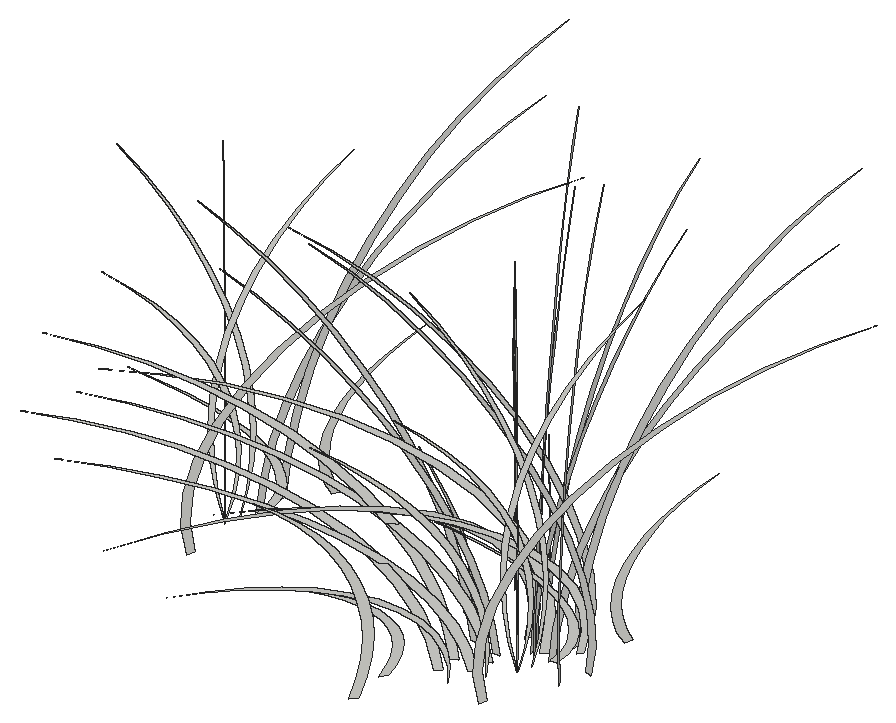
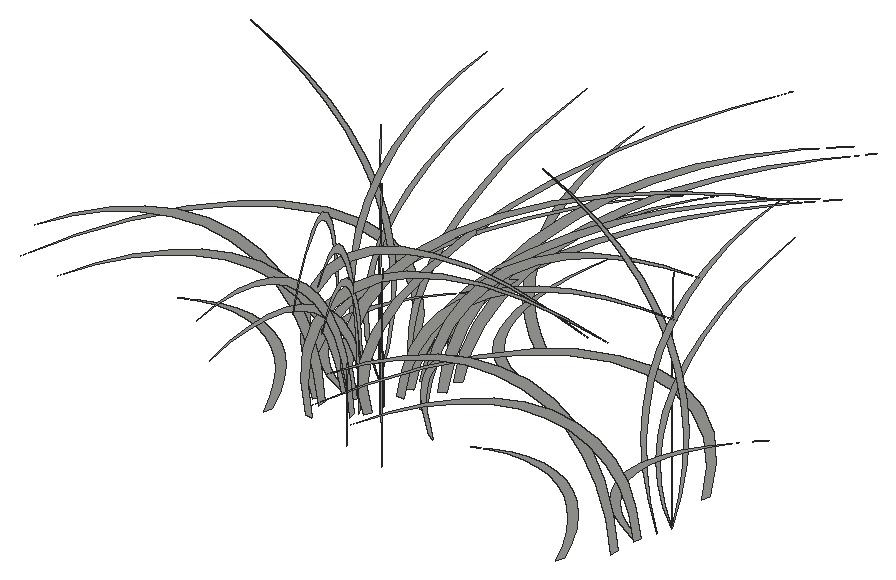
# SketchUp Ruby script. Lengths in inches.
U = 1.inch
M = Sketchup.active_model
def pt(a) = Geom::Point3d.new(a.map { |v| v * U })
def face(e, loops, mat)
  f = e.add_face(loops[0].map { |a| pt(a) })
  loops[1..].each { |l| e.add_face(l.map { |a| pt(a) }).erase! }
  f.material = f.back_material = mat if mat
  f
end
# faces: each face lists its corners as indices into pts; further lists are holes
def faces(e, pts, list, mat = nil) = list.each { |f| face(e, (f[0].is_a?(Array) ? f : [f]).map { |l| l.map { |i| pts[i] } }, mat) }
# xy, xz, yz: faces in a plane at the given z, y or x. An outline is a flat list of corners, or four numbers for a rectangle; further outlines are holes
def ring(l) = l.size == 4 ? [[l[0], l[1]], [l[2], l[1]], [l[2], l[3]], [l[0], l[3]]] : l.each_slice(2).to_a
def flat(e, list, mat, &to3) = list.each { |f| face(e, (f[0].is_a?(Array) ? f : [f]).map { |l| ring(l).map { |u, v| to3.(u, v) } }, mat) }
def xy(e, z, list, mat = nil) = flat(e, list, mat) { |x, y| [x, y, z] }
def xz(e, y, list, mat = nil) = flat(e, list, mat) { |x, z| [x, y, z] }
def yz(e, x, list, mat = nil) = flat(e, list, mat) { |y, z| [x, y, z] }
def lines(e, pts, list) = list.each { |a, b| e.add_line(pt(pts[a]), pt(pts[b])) }
# prism: a flat outline (further loops are holes) pulled along v
def prism(e, loops, v, mat = nil)
  f = face(e, loops, mat); d = Geom::Vector3d.new(v.map { |x| x * U })
  f.pushpull(f.normal.samedirection?(d) ? d.length : -d.length)
end
def box(e, o, s, mat = nil) = prism(e, [[o, [o[0] + s[0], o[1], o[2]], [o[0] + s[0], o[1] + s[1], o[2]], [o[0], o[1] + s[1], o[2]]]], [0, 0, s[2]], mat)
def at(x, y, z, deg = 0) = Geom::Transformation.translation(pt([x, y, z])) * Geom::Transformation.rotation(ORIGIN, Z_AXIS, deg.degrees)
def axes(o, x, y, z) = Geom::Transformation.new([*x, 0, *y, 0, *z, 0, *pt(o).to_a, 1])
def part(name) = M.definitions.add(name)
# library, detail: a bought-in or finely detailed component or shape, given as its bounding box
def library(name, o, s) = part(name).tap { |d| box(d.entities, o, s) }
def detail(e, o, s) = box(e.add_group.entities, o, s)
def put(e, d, t, mat = nil) = e.add_instance(d, t).tap { |i| i.material = mat if mat }
def group(e, t, mat = nil) = e.add_group.tap { |g| g.transformation = t; g.material = mat if mat }.entities
root = M.entities
g1 = group(root,at(499.02,261.86,0))
p = [[-0.89,-0.32,0],[-0.4,-0.14,1.97],[-0.1,-0.04,3.96],[0,0,5.95],[-0.1,-0.03,7.95],[-0.39,-0.14,9.9375],
  [-0.89,-0.3125,11.91],[-1.57,-0.56,13.85],[-2.45,-0.87,15.76],[-3.52,-1.25,17.63],[-4.77,-1.6875,19.44],[-6.19,-2.19,21.2],
  [-7.79,-2.76,22.89],[-6.29,-2.23,21.17],[-4.94,-1.75,19.4],[-3.76,-1.33,17.58],[-2.74,-0.97,15.71],[-1.89,-0.67,13.8],
  [-1.22,-0.43,11.86],[-0.72,-0.25,9.9],[-0.4,-0.14,7.93],[-0.25,-0.09,5.94],[-0.29,-0.1,3.95],[-0.5,-0.18,1.97]]
faces(g1,p,[[0,1,2,3,4,5,6,7,8,9,10,11,12,13,14,15,16,17,18,19,20,21,22,23]])
g2 = group(root,at(500.125,263.22,0))
p = [[-9.01,-2.98,7.88],[-7.3,-2.41,7.38],[-5.75,-1.9,6.83],[-4.38,-1.45,6.24],[-3.2,-1.06,5.62],[-2.23,-0.74,4.96],
  [-1.47,-0.49,4.27],[-0.92,-0.31,3.57],[-0.61,-0.2,2.86],[-0.51,-0.17,2.13],[-0.65,-0.21,1.41],[-1.01,-0.33,0.7],
  [-1.6,-0.53,0],[-1.21,-0.4,0],[-0.54,-0.18,0.69],[-0.12,-0.04,1.4],[0.06,0.02,2.13],[-0.02,-0.01,2.85],
  [-0.35,-0.11,3.58],[-0.92,-0.3,4.29],[-1.73,-0.57,4.98],[-2.78,-0.92,5.64],[-4.05,-1.34,6.27],[-5.52,-1.82,6.86],
  [-7.18,-2.375,7.4]]
faces(g2,p,[[0,1,2,3,4,5,6,7,8,9,10,11,12,13,14,15,16,17,18,19,20,21,22,23,24]])
g3 = group(root,at(498.46,259.83,0))
p = [[-0.6,0.73,0],[-0.27,0.33,1.77],[-0.07,0.08,3.57],[0,0,5.36],[-0.07,0.08,7.16],[-0.27,0.32,8.95],
  [-0.6,0.73,10.73],[-1.06,1.29,12.48],[-1.65,2.01,14.2],[-2.37,2.88,15.88],[-3.21,3.91,17.52],[-4.17,5.08,19.1],
  [-5.25,6.39,20.625],[-4.23,5.15,19.08],[-3.33,4.05,17.48],[-2.53,3.08,15.83],[-1.84,2.25,14.15],[-1.27,1.55,12.43],
  [-0.82,1,10.6875],[-0.48,0.59,8.92],[-0.27,0.32,7.14],[-0.17,0.21,5.35],[-0.19,0.24,3.5625],[-0.34,0.41,1.78]]
faces(g3,p,[[0,1,2,3,4,5,6,7,8,9,10,11,12,13,14,15,16,17,18,19,20,21,22,23]])
g4 = group(root,at(498.38,261.36,0))
p = [[-0.52,-0.79,0],[-0.23,-0.35,1.51],[-0.06,-0.09,3.03],[0,0,4.56],[-0.06,-0.09,6.09],[-0.23,-0.35,7.61],
  [-0.52,-0.79,9.12],[-0.92,-1.39,10.61],[-1.43,-2.17,12.07],[-2.05,-3.12,13.5],[-2.78,-4.23,14.89],[-3.61,-5.49,16.24],
  [-4.54,-6.91,17.53],[-3.66,-5.57,16.21],[-2.88,-4.38,14.86],[-2.1875,-3.33,13.46],[-1.6,-2.43,12.03],[-1.1,-1.68,10.57],
  [-0.71,-1.08,9.08],[-0.42,-0.64,7.58],[-0.23,-0.35,6.07],[-0.15,-0.22,4.55],[-0.17,-0.25,3.03],[-0.29,-0.44,1.51]]
faces(g4,p,[[0,1,2,3,4,5,6,7,8,9,10,11,12,13,14,15,16,17,18,19,20,21,22,23]])
g5 = group(root,at(498.48,262.59,0))
p = [[1.63,20.71,16.73],[1.875,23.84,17.17],[1.64,20.8125,16.64],[1.41,17.89,15.9],[1.1875,15.1,14.96],[0.98,12.48,13.84],
  [0.79,10.06,12.54],[0.62,7.86,11.08],[0.47,5.91,9.48],[0.33,4.23,7.76],[0.22,2.84,5.92],[0.14,1.75,4.01],
  [0.08,0.98,2.02],[0.04,0.54,0],[0,0,0],[0.03,0.36,2.07],[0.09,1.09,4.1],[0.17,2.15,6.07],
  [0.28,3.55,7.94],[0.41,5.27,9.7],[0.57,7.28,11.33],[0.75,9.55,12.79],[0.95,12.07,14.08],[1.16,14.79,15.17],
  [1.39,17.68,16.0625]]
faces(g5,p,[[0,1,2,3,4,5,6,7,8,9,10,11,12,13,14,15,16,17,18,19,20,21,22,23,24]])
g6 = group(root,at(498.63,264.51,0))
p = [[1.63,20.71,20.75],[1.875,23.84,21.3],[1.64,20.8125,20.63],[1.41,17.89,19.72],[1.1875,15.1,18.55],[0.98,12.48,17.16],
  [0.79,10.06,15.55],[0.62,7.86,13.74],[0.47,5.91,11.76],[0.33,4.23,9.62],[0.22,2.84,7.35],[0.14,1.75,4.97],
  [0.08,0.98,2.51],[0.04,0.54,0],[0,0,0],[0.03,0.36,2.57],[0.09,1.09,5.09],[0.17,2.15,7.53],
  [0.28,3.55,9.85],[0.41,5.27,12.03],[0.57,7.28,14.04],[0.75,9.55,15.86],[0.95,12.07,17.46],[1.16,14.79,18.82],
  [1.39,17.68,19.92]]
faces(g6,p,[[0,1,2,3,4,5,6,7,8,9,10,11,12,13,14,15,16,17,18,19,20,21,22,23,24]])
g7 = group(root,at(497.1875,259.9,0))
p = [[0.67,0.67,0],[0.3,0.3,2.04],[0.08,0.08,4.1],[0,0,6.17],[0.07,0.07,8.23],[0.3,0.3,10.29],
  [0.66,0.66,12.33],[1.18,1.18,14.34],[1.84,1.84,16.32],[2.64,2.64,18.26],[3.58,3.58,20.14],[4.65,4.65,21.96],
  [5.84,5.84,23.71],[4.72,4.72,21.93],[3.71,3.71,20.09],[2.82,2.82,18.2],[2.05,2.05,16.26],[1.42,1.42,14.29],
  [0.91,0.91,12.29],[0.54,0.54,10.26],[0.3,0.3,8.21],[0.1875,0.1875,6.15],[0.22,0.22,4.09],[0.375,0.375,2.04]]
faces(g7,p,[[0,1,2,3,4,5,6,7,8,9,10,11,12,13,14,15,16,17,18,19,20,21,22,23]])
g8 = group(root,at(500.18,266.11,0))
p = [[2.34,6.79,9.0625],[1.91,5.55,8.49],[1.52,4.43,7.85],[1.18,3.44,7.18],[0.89,2.58,6.45],[0.65,1.88,5.7],
  [0.46,1.33,4.91],[0.32,0.93,4.1],[0.24,0.7,3.28],[0.22,0.64,2.45],[0.25,0.74,1.625],[0.34,1,0.8],
  [0.49,1.42,0],[0.3,0.875,0],[0.14,0.4,0.81],[0.04,0.11,1.65],[0,0,2.49],[0.03,0.07,3.34],
  [0.11,0.33,4.17],[0.27,0.77,4.99],[0.48,1.38,5.79],[0.75,2.17,6.54],[1.07,3.11,7.26],[1.45,4.2,7.92],
  [1.87,5.43,8.52]]
faces(g8,p,[[0,1,2,3,4,5,6,7,8,9,10,11,12,13,14,15,16,17,18,19,20,21,22,23,24]])
g9 = group(root,at(498.33,255.96,0))
p = [[0.26,0.96,0],[0.11,0.43,0],[0,0,2.01],[0.05,0.17,4.04],[0.25,0.9375,6.02],[0.62,2.28,7.92],
  [1.125,4.16,9.68],[1.76,6.54,11.26],[2.52,9.35,12.62],[3.38,12.53,13.73],[4.32,16,14.5625],[5.31,19.67,15.09],
  [6.33,23.45,15.31],[7.35,27.24,15.2],[6.35,23.52,15.22],[5.35,19.83,14.94],[4.39,16.27,14.37],[3.48,12.91,13.51],
  [2.65,9.83,12.39],[1.92,7.11,11.04],[1.29,4.8,9.48],[0.8,2.96,7.75],[0.44,1.63,5.9],[0.23,0.84,3.96],
  [0.17,0.62,1.98]]
faces(g9,p,[[0,1,2,3,4,5,6,7,8,9,10,11,12,13,14,15,16,17,18,19,20,21,22,23,24]])
g10 = group(root,at(517.58,258.66,0))
p = [[-20.46,3.64,18.05],[-23.54,4.19,18.53],[-20.55,3.66,17.95],[-17.67,3.15,17.15],[-14.91,2.66,16.14],[-12.33,2.2,14.93],
  [-9.93,1.77,13.53],[-7.76,1.38,11.96],[-5.84,1.04,10.23],[-4.18,0.74,8.37],[-2.8,0.5,6.39],[-1.73,0.31,4.32],
  [-0.97,0.17,2.18],[-0.53,0.09,0],[0,0,0],[-0.36,0.0625,2.23],[-1.07,0.19,4.43],[-2.125,0.38,6.55],
  [-3.51,0.625,8.57],[-5.2,0.93,10.47],[-7.1875,1.28,12.22],[-9.43,1.68,13.8],[-11.92,2.125,15.1875],[-14.61,2.6,16.37],
  [-17.46,3.11,17.33]]
faces(g10,p,[[0,1,2,3,4,5,6,7,8,9,10,11,12,13,14,15,16,17,18,19,20,21,22,23,24]])
g11 = group(root,at(517.97,256.5625,0))
p = [[-18.45,-9.5625,18.05],[-21.23,-11,18.53],[-18.53,-9.61,17.95],[-15.93,-8.26,17.15],[-13.45,-6.97,16.14],[-11.12,-5.76,14.93],
  [-8.96,-4.64,13.53],[-7,-3.63,11.96],[-5.26,-2.73,10.23],[-3.77,-1.95,8.37],[-2.53,-1.3125,6.39],[-1.5625,-0.81,4.32],
  [-0.875,-0.45,2.18],[-0.48,-0.25,0],[0,0,0],[-0.32,-0.17,2.23],[-0.97,-0.5,4.43],[-1.92,-0.99,6.55],
  [-3.16,-1.64,8.57],[-4.69,-2.43,10.47],[-6.48,-3.36,12.22],[-8.51,-4.41,13.8],[-10.75,-5.57,15.1875],[-13.17,-6.83,16.37],
  [-15.75,-8.16,17.33]]
faces(g11,p,[[0,1,2,3,4,5,6,7,8,9,10,11,12,13,14,15,16,17,18,19,20,21,22,23,24]])
g12 = group(root,at(517.97,256.5625,0))
p = [[-18.45,-9.5625,18.05],[-21.23,-11,18.53],[-18.53,-9.61,17.95],[-15.93,-8.26,17.15],[-13.45,-6.97,16.14],[-11.12,-5.76,14.93],
  [-8.96,-4.64,13.53],[-7,-3.63,11.96],[-5.26,-2.73,10.23],[-3.77,-1.95,8.37],[-2.53,-1.3125,6.39],[-1.5625,-0.81,4.32],
  [-0.875,-0.45,2.18],[-0.48,-0.25,0],[0,0,0],[-0.32,-0.17,2.23],[-0.97,-0.5,4.43],[-1.92,-0.99,6.55],
  [-3.16,-1.64,8.57],[-4.69,-2.43,10.47],[-6.48,-3.36,12.22],[-8.51,-4.41,13.8],[-10.75,-5.57,15.1875],[-13.17,-6.83,16.37],
  [-15.75,-8.16,17.33]]
faces(g12,p,[[0,1,2,3,4,5,6,7,8,9,10,11,12,13,14,15,16,17,18,19,20,21,22,23,24]])
g13 = group(root,at(519.48,258.32,0))
p = [[-20.46,3.64,14.56],[-23.54,4.19,14.94],[-20.55,3.66,14.48],[-17.67,3.15,13.83],[-14.91,2.66,13.02],[-12.33,2.2,12.04],
  [-9.93,1.77,10.91],[-7.76,1.38,9.64],[-5.84,1.04,8.25],[-4.18,0.74,6.75],[-2.8,0.5,5.15],[-1.73,0.31,3.49],
  [-0.97,0.17,1.76],[-0.53,0.09,0],[0,0,0],[-0.36,0.0625,1.8],[-1.07,0.19,3.57],[-2.125,0.38,5.28],
  [-3.51,0.625,6.91],[-5.2,0.93,8.44],[-7.1875,1.28,9.85],[-9.43,1.68,11.13],[-11.92,2.125,12.25],[-14.61,2.6,13.2],
  [-17.46,3.11,13.97]]
faces(g13,p,[[0,1,2,3,4,5,6,7,8,9,10,11,12,13,14,15,16,17,18,19,20,21,22,23,24]])
g14 = group(root,at(518.01,255.07,0))
p = [[-17.17,-11.7,15.34],[-19.76,-13.47,15.75],[-17.25,-11.76,15.26],[-14.83,-10.11,14.58],[-12.52,-8.53,13.72],[-10.35,-7.05,12.69],
  [-8.34,-5.68,11.5],[-6.52,-4.44,10.16],[-4.9,-3.34,8.7],[-3.51,-2.39,7.11],[-2.35,-1.6,5.43],[-1.45,-0.99,3.67],
  [-0.82,-0.56,1.86],[-0.45,-0.3,0],[0,0,0],[-0.3,-0.21,1.9],[-0.9,-0.61,3.76],[-1.78,-1.22,5.57],
  [-2.95,-2.01,7.28],[-4.37,-2.98,8.9],[-6.03,-4.11,10.39],[-7.92,-5.4,11.73],[-10,-6.82,12.91],[-12.26,-8.36,13.91],
  [-14.66,-9.99,14.73]]
faces(g14,p,[[0,1,2,3,4,5,6,7,8,9,10,11,12,13,14,15,16,17,18,19,20,21,22,23,24]])
g15 = group(root,at(519.6875,257.45,0))
p = [[-18.45,-9.5625,14.56],[-21.23,-11,14.94],[-18.53,-9.61,14.48],[-15.93,-8.26,13.83],[-13.45,-6.97,13.02],[-11.12,-5.76,12.04],
  [-8.96,-4.64,10.91],[-7,-3.63,9.64],[-5.26,-2.73,8.25],[-3.77,-1.95,6.75],[-2.53,-1.3125,5.15],[-1.5625,-0.81,3.49],
  [-0.875,-0.45,1.76],[-0.48,-0.25,0],[0,0,0],[-0.32,-0.17,1.8],[-0.97,-0.5,3.57],[-1.92,-0.99,5.28],
  [-3.16,-1.64,6.91],[-4.69,-2.43,8.44],[-6.48,-3.36,9.85],[-8.51,-4.41,11.13],[-10.75,-5.57,12.25],[-13.17,-6.83,13.2],
  [-15.75,-8.16,13.97]]
faces(g15,p,[[0,1,2,3,4,5,6,7,8,9,10,11,12,13,14,15,16,17,18,19,20,21,22,23,24]])
g16 = group(root,at(519.6875,257.45,0))
p = [[-18.45,-9.5625,14.56],[-21.23,-11,14.94],[-18.53,-9.61,14.48],[-15.93,-8.26,13.83],[-13.45,-6.97,13.02],[-11.12,-5.76,12.04],
  [-8.96,-4.64,10.91],[-7,-3.63,9.64],[-5.26,-2.73,8.25],[-3.77,-1.95,6.75],[-2.53,-1.3125,5.15],[-1.5625,-0.81,3.49],
  [-0.875,-0.45,1.76],[-0.48,-0.25,0],[0,0,0],[-0.32,-0.17,1.8],[-0.97,-0.5,3.57],[-1.92,-0.99,5.28],
  [-3.16,-1.64,6.91],[-4.69,-2.43,8.44],[-6.48,-3.36,9.85],[-8.51,-4.41,11.13],[-10.75,-5.57,12.25],[-13.17,-6.83,13.2],
  [-15.75,-8.16,13.97]]
faces(g16,p,[[0,1,2,3,4,5,6,7,8,9,10,11,12,13,14,15,16,17,18,19,20,21,22,23,24]])
g17 = group(root,at(522.55,263.17,0))
p = [[-0.91,0.16,0],[-0.4,0.07,0],[0,0,2.0625],[-0.16,0.03,4.13],[-0.89,0.16,6.16],[-2.17,0.39,8.1],
  [-3.95,0.7,9.91],[-6.21,1.11,11.52],[-8.88,1.58,12.92],[-11.91,2.12,14.05],[-15.2,2.71,14.9],[-18.68,3.33,15.45],
  [-22.27,3.97,15.67],[-25.88,4.61,15.5625],[-22.34,3.98,15.58],[-18.84,3.36,15.29],[-15.45,2.75,14.71],[-12.26,2.18,13.83],
  [-9.34,1.66,12.68],[-6.75,1.2,11.3],[-4.56,0.8125,9.7],[-2.81,0.5,7.9375],[-1.55,0.28,6.04],[-0.8,0.14,4.05],
  [-0.59,0.1,2.02]]
faces(g17,p,[[0,1,2,3,4,5,6,7,8,9,10,11,12,13,14,15,16,17,18,19,20,21,22,23,24]])
g18 = group(root,at(522.55,263.17,0))
p = [[-0.91,0.16,0],[-0.4,0.07,0],[0,0,2.0625],[-0.16,0.03,4.13],[-0.89,0.16,6.16],[-2.17,0.39,8.1],
  [-3.95,0.7,9.91],[-6.21,1.11,11.52],[-8.88,1.58,12.92],[-11.91,2.12,14.05],[-15.2,2.71,14.9],[-18.68,3.33,15.45],
  [-22.27,3.97,15.67],[-25.88,4.61,15.5625],[-22.34,3.98,15.58],[-18.84,3.36,15.29],[-15.45,2.75,14.71],[-12.26,2.18,13.83],
  [-9.34,1.66,12.68],[-6.75,1.2,11.3],[-4.56,0.8125,9.7],[-2.81,0.5,7.9375],[-1.55,0.28,6.04],[-0.8,0.14,4.05],
  [-0.59,0.1,2.02]]
faces(g18,p,[[0,1,2,3,4,5,6,7,8,9,10,11,12,13,14,15,16,17,18,19,20,21,22,23,24]])
g19 = group(root,at(519.61,256.16,0))
p = [[-17.17,-11.7,12.375],[-19.76,-13.47,12.7],[-17.25,-11.76,12.31],[-14.83,-10.11,11.76],[-12.52,-8.53,11.07],[-10.35,-7.05,10.23],
  [-8.34,-5.68,9.27],[-6.52,-4.44,8.2],[-4.9,-3.34,7.01],[-3.51,-2.39,5.74],[-2.35,-1.6,4.38],[-1.45,-0.99,2.96],
  [-0.82,-0.56,1.5],[-0.45,-0.3,0],[0,0,0],[-0.3,-0.21,1.53],[-0.9,-0.61,3.03],[-1.78,-1.22,4.49],
  [-2.95,-2.01,5.875],[-4.37,-2.98,7.18],[-6.03,-4.11,8.375],[-7.92,-5.4,9.46],[-10,-6.82,10.41],[-12.26,-8.36,11.22],
  [-14.66,-9.99,11.88]]
faces(g19,p,[[0,1,2,3,4,5,6,7,8,9,10,11,12,13,14,15,16,17,18,19,20,21,22,23,24]])
g20 = group(root,at(521.8125,260.48,0))
p = [[-0.82,-0.43,0],[-0.36,-0.1875,0],[0,0,2.0625],[-0.15,-0.08,4.13],[-0.8,-0.42,6.16],[-1.95,-1.01,8.1],
  [-3.57,-1.85,9.91],[-5.6,-2.9,11.52],[-8.01,-4.15,12.92],[-10.74,-5.57,14.05],[-13.71,-7.1,14.9],[-16.85,-8.73,15.45],
  [-20.09,-10.41,15.67],[-23.34,-12.1,15.5625],[-20.15,-10.44,15.58],[-16.99,-8.81,15.29],[-13.9375,-7.22,14.71],[-11.06,-5.73,13.83],
  [-8.42,-4.37,12.68],[-6.09,-3.16,11.3],[-4.11,-2.13,9.7],[-2.53,-1.3125,7.9375],[-1.4,-0.72,6.04],[-0.72,-0.375,4.05],
  [-0.53,-0.27,2.02]]
faces(g20,p,[[0,1,2,3,4,5,6,7,8,9,10,11,12,13,14,15,16,17,18,19,20,21,22,23,24]])
g21 = group(root,at(525.41,259.61,0))
p = [[-0.95,0.28,0],[-0.42,0.125,0],[0,0,2.01],[-0.17,0.05,4.04],[-0.93,0.27,6.02],[-2.27,0.66,7.92],
  [-4.14,1.21,9.68],[-6.5,1.9,11.26],[-9.3,2.72,12.62],[-12.46,3.64,13.73],[-15.91,4.65,14.5625],[-19.55,5.72,15.09],
  [-23.3125,6.82,15.31],[-27.08,7.92,15.2],[-23.38,6.84,15.22],[-19.72,5.77,14.94],[-16.17,4.73,14.37],[-12.83,3.75,13.51],
  [-9.77,2.86,12.39],[-7.0625,2.07,11.04],[-4.77,1.39,9.48],[-2.94,0.86,7.75],[-1.62,0.47,5.9],[-0.84,0.25,3.96],
  [-0.61,0.18,1.98]]
faces(g21,p,[[0,1,2,3,4,5,6,7,8,9,10,11,12,13,14,15,16,17,18,19,20,21,22,23,24]])
g22 = group(root,at(516.14,260.36,0))
p = [[-6.53,2.99,7.88],[-5.33,2.44,7.38],[-4.26,1.95,6.83],[-3.3,1.51,6.24],[-2.48,1.14,5.62],[-1.81,0.83,4.96],
  [-1.28,0.58,4.27],[-0.9,0.41,3.57],[-0.68,0.31,2.86],[-0.61,0.28,2.13],[-0.71,0.32,1.41],[-0.96,0.4375,0.7],
  [-1.37,0.625,0],[-0.84,0.38,0],[-0.39,0.18,0.71],[-0.11,0.05,1.43],[0,0,2.17],[-0.07,0.03,2.9],
  [-0.32,0.15,3.63],[-0.74,0.34,4.34],[-1.33,0.61,5.03],[-2.08,0.95,5.69],[-2.99,1.37,6.3125],[-4.04,1.85,6.89],
  [-5.22,2.39,7.41]]
faces(g22,p,[[0,1,2,3,4,5,6,7,8,9,10,11,12,13,14,15,16,17,18,19,20,21,22,23,24]])
g23 = group(root,at(518.9,260.59,0))
p = [[-10.66,12.98,9.9],[-9.23,11.23,9.83],[-7.82,9.52,9.59],[-6.46,7.86,9.18],[-5.18,6.3,8.61],[-3.99,4.86,7.88],
  [-2.93,3.57,7.02],[-2.02,2.46,6.03],[-1.27,1.54,4.95],[-0.6875,0.84,3.78],[-0.29,0.36,2.55],[-0.1,0.12,1.28],
  [-0.09,0.12,0],[0,0,1.3],[-0.125,0.15,2.61],[-0.47,0.57,3.875],[-1.02,1.24,5.09],[-1.77,2.15,6.21],
  [-2.69,3.28,7.22],[-3.78,4.6,8.1],[-5,6.09,8.82],[-6.33,7.71,9.37],[-7.74,9.43,9.74],[-9.2,11.19,9.92]]
faces(g23,p,[[0,1,2,3,4,5,6,7,8,9,10,11,12,13,14,15,16,17,18,19,20,21,22,23]])
g24 = group(root,at(520.16,260.86,0))
p = [[-11.32,17.43,20.75],[-13.02,20.05,21.3],[-11.37,17.51,20.63],[-9.77,15.05,19.72],[-8.25,12.7,18.55],[-6.82,10.5,17.16],
  [-5.5,8.46,15.55],[-4.29,6.61,13.74],[-3.23,4.97,11.76],[-2.3125,3.56,9.62],[-1.55,2.39,7.35],[-0.96,1.47,4.97],
  [-0.54,0.83,2.51],[-0.29,0.45,0],[0,0,0],[-0.2,0.31,2.57],[-0.59,0.91,5.09],[-1.18,1.8125,7.53],
  [-1.94,2.99,9.85],[-2.88,4.43,12.03],[-3.98,6.12,14.04],[-5.22,8.04,15.86],[-6.59,10.15,17.46],[-8.08,12.44,18.82],
  [-9.66,14.88,19.92]]
faces(g24,p,[[0,1,2,3,4,5,6,7,8,9,10,11,12,13,14,15,16,17,18,19,20,21,22,23,24]])
g25 = group(root,at(516.03,264.08,0))
p = [[-4.56,5.55,16.02],[-3.72,4.53,15.01],[-2.97,3.62,13.89],[-2.31,2.81,12.69],[-1.73,2.11,11.42],[-1.26,1.54,10.08],
  [-0.89,1.09,8.6875],[-0.63,0.76,7.26],[-0.47,0.58,5.8],[-0.43,0.52,4.34],[-0.49,0.6,2.87],[-0.67,0.81,1.42],
  [-0.95,1.16,0],[-0.59,0.71,0],[-0.27,0.33,1.44],[-0.07,0.09,2.92],[0,0,4.41],[-0.05,0.0625,5.9],
  [-0.22,0.27,7.38],[-0.52,0.63,8.83],[-0.93,1.13,10.23],[-1.45,1.77,11.57],[-2.09,2.54,12.83],[-2.82,3.43,14.01],
  [-3.65,4.44,15.07]]
faces(g25,p,[[0,1,2,3,4,5,6,7,8,9,10,11,12,13,14,15,16,17,18,19,20,21,22,23,24]])
g26 = group(root,at(516.03,264.08,0))
p = [[-4.56,5.55,16.02],[-3.72,4.53,15.01],[-2.97,3.62,13.89],[-2.31,2.81,12.69],[-1.73,2.11,11.42],[-1.26,1.54,10.08],
  [-0.89,1.09,8.6875],[-0.63,0.76,7.26],[-0.47,0.58,5.8],[-0.43,0.52,4.34],[-0.49,0.6,2.87],[-0.67,0.81,1.42],
  [-0.95,1.16,0],[-0.59,0.71,0],[-0.27,0.33,1.44],[-0.07,0.09,2.92],[0,0,4.41],[-0.05,0.0625,5.9],
  [-0.22,0.27,7.38],[-0.52,0.63,8.83],[-0.93,1.13,10.23],[-1.45,1.77,11.57],[-2.09,2.54,12.83],[-2.82,3.43,14.01],
  [-3.65,4.44,15.07]]
faces(g26,p,[[0,1,2,3,4,5,6,7,8,9,10,11,12,13,14,15,16,17,18,19,20,21,22,23,24]])
g27 = group(root,at(519.73,261.66,0))
p = [[-0.37,-0.92,0],[-0.16,-0.41,0],[0,0,1.75],[-0.07,-0.17,3.51],[-0.36,-0.9,5.24],[-0.88,-2.19,6.89],
  [-1.61,-4,8.42],[-2.53,-6.28,9.8],[-3.61,-8.99,10.98],[-4.84,-12.04,11.95],[-6.18,-15.375,12.67],[-7.6,-18.9,13.13],
  [-9.06,-22.53,13.32],[-10.53,-26.18,13.23],[-9.09,-22.6,13.25],[-7.66,-19.06,13],[-6.29,-15.63,12.5],[-4.99,-12.41,11.75],
  [-3.8,-9.45,10.78],[-2.75,-6.83,9.6],[-1.85,-4.61,8.25],[-1.14,-2.84,6.75],[-0.63,-1.57,5.13],[-0.33,-0.8125,3.44],
  [-0.24,-0.59,1.72]]
faces(g27,p,[[0,1,2,3,4,5,6,7,8,9,10,11,12,13,14,15,16,17,18,19,20,21,22,23,24]])
g28 = group(root,at(516.47,253.48,0))
p = [[-3.94,-6,6.7],[-3.22,-4.9,6.27],[-2.57,-3.91,5.81],[-2,-3.04,5.31],[-1.5,-2.28,4.77],[-1.09,-1.66,4.21],
  [-0.77,-1.17,3.63],[-0.54,-0.83,3.03],[-0.41,-0.62,2.43],[-0.37,-0.5625,1.8125],[-0.43,-0.65,1.2],[-0.58,-0.88,0.59],
  [-0.83,-1.26,0],[-0.51,-0.77,0],[-0.23,-0.36,0.6],[-0.0625,-0.1,1.22],[0,0,1.84],[-0.04,-0.07,2.47],
  [-0.19,-0.29,3.09],[-0.45,-0.68,3.69],[-0.8,-1.22,4.28],[-1.26,-1.91,4.84],[-1.81,-2.75,5.37],[-2.44,-3.71,5.86],
  [-3.16,-4.8,6.3]]
faces(g28,p,[[0,1,2,3,4,5,6,7,8,9,10,11,12,13,14,15,16,17,18,19,20,21,22,23,24]])
g29 = group(root,at(519.24,254.17,0))
p = [[-9.23,-14.04,8.41],[-7.99,-12.15,8.36],[-6.77,-10.29,8.15],[-5.59,-8.5,7.8],[-4.48,-6.8125,7.32],[-3.46,-5.26,6.7],
  [-2.54,-3.86,5.97],[-1.75,-2.66,5.13],[-1.09,-1.67,4.2],[-0.59,-0.9,3.21],[-0.25,-0.39,2.16],[-0.08,-0.125,1.09],
  [-0.08,-0.125,0],[0,0,1.11],[-0.11,-0.16,2.21],[-0.4,-0.61,3.29],[-0.88,-1.34,4.32],[-1.53,-2.33,5.28],
  [-2.33,-3.55,6.14],[-3.27,-4.98,6.88],[-4.33,-6.59,7.5],[-5.48,-8.34,7.97],[-6.7,-10.19,8.28],[-7.96,-12.11,8.43]]
faces(g29,p,[[0,1,2,3,4,5,6,7,8,9,10,11,12,13,14,15,16,17,18,19,20,21,22,23]])
g30 = group(root,at(521.21,259.24,0))
p = [[-11.32,17.43,16.73],[-13.02,20.05,17.17],[-11.37,17.51,16.64],[-9.77,15.05,15.9],[-8.25,12.7,14.96],[-6.82,10.5,13.84],
  [-5.5,8.46,12.54],[-4.29,6.61,11.08],[-3.23,4.97,9.48],[-2.3125,3.56,7.76],[-1.55,2.39,5.92],[-0.96,1.47,4.01],
  [-0.54,0.83,2.02],[-0.29,0.45,0],[0,0,0],[-0.2,0.31,2.07],[-0.59,0.91,4.1],[-1.18,1.8125,6.07],
  [-1.94,2.99,7.94],[-2.88,4.43,9.7],[-3.98,6.12,11.33],[-5.22,8.04,12.79],[-6.59,10.15,14.08],[-8.08,12.44,15.17],
  [-9.66,14.88,16.0625]]
faces(g30,p,[[0,1,2,3,4,5,6,7,8,9,10,11,12,13,14,15,16,17,18,19,20,21,22,23,24]])
g31 = group(root,at(516.76,250.4,0))
p = [[-3.94,-6,13.62],[-3.22,-4.9,12.76],[-2.57,-3.91,11.81],[-2,-3.04,10.79],[-1.5,-2.28,9.7],[-1.09,-1.66,8.57],
  [-0.77,-1.17,7.38],[-0.54,-0.83,6.17],[-0.41,-0.62,4.93],[-0.37,-0.5625,3.6875],[-0.43,-0.65,2.44],[-0.58,-0.88,1.21],
  [-0.83,-1.26,0],[-0.51,-0.77,0],[-0.23,-0.36,1.22],[-0.0625,-0.1,2.48],[0,0,3.75],[-0.04,-0.07,5.02],
  [-0.19,-0.29,6.28],[-0.45,-0.68,7.51],[-0.8,-1.22,8.7],[-1.26,-1.91,9.84],[-1.81,-2.75,10.91],[-2.44,-3.71,11.9],
  [-3.16,-4.8,12.8125]]
faces(g31,p,[[0,1,2,3,4,5,6,7,8,9,10,11,12,13,14,15,16,17,18,19,20,21,22,23,24]])
g32 = group(root,at(523.23,261.82,0))
p = [[-0.5,-0.57,0],[-0.22,-0.25,0],[0,0,1.46],[-0.09,-0.1,2.93],[-0.49,-0.56,4.375],[-1.19,-1.35,5.75],
  [-2.17,-2.47,7.03],[-3.41,-3.89,8.18],[-4.88,-5.56,9.17],[-6.54,-7.45,9.98],[-8.36,-9.51,10.58],[-10.27,-11.69,10.97],
  [-12.24,-13.9375,11.125],[-14.23,-16.19,11.05],[-12.28,-13.98,11.0625],[-10.36,-11.79,10.86],[-8.5,-9.67,10.44],[-6.74,-7.67,9.82],
  [-5.13,-5.84,9.01],[-3.71,-4.22,8.02],[-2.51,-2.85,6.89],[-1.54,-1.76,5.64],[-0.85,-0.97,4.29],[-0.44,-0.5,2.88],
  [-0.32,-0.37,1.4375]]
faces(g32,p,[[0,1,2,3,4,5,6,7,8,9,10,11,12,13,14,15,16,17,18,19,20,21,22,23,24]])
g33 = group(root,at(523.23,261.82,0))
p = [[-0.5,-0.57,0],[-0.22,-0.25,0],[0,0,1.46],[-0.09,-0.1,2.93],[-0.49,-0.56,4.375],[-1.19,-1.35,5.75],
  [-2.17,-2.47,7.03],[-3.41,-3.89,8.18],[-4.88,-5.56,9.17],[-6.54,-7.45,9.98],[-8.36,-9.51,10.58],[-10.27,-11.69,10.97],
  [-12.24,-13.9375,11.125],[-14.23,-16.19,11.05],[-12.28,-13.98,11.0625],[-10.36,-11.79,10.86],[-8.5,-9.67,10.44],[-6.74,-7.67,9.82],
  [-5.13,-5.84,9.01],[-3.71,-4.22,8.02],[-2.51,-2.85,6.89],[-1.54,-1.76,5.64],[-0.85,-0.97,4.29],[-0.44,-0.5,2.88],
  [-0.32,-0.37,1.4375]]
faces(g33,p,[[0,1,2,3,4,5,6,7,8,9,10,11,12,13,14,15,16,17,18,19,20,21,22,23,24]])
g34 = group(root,at(520.12,261.49,0))
p = [[-6.07,19.87,18.05],[-6.99,22.87,18.53],[-6.1,19.96,17.95],[-5.25,17.16,17.15],[-4.43,14.49,16.14],[-3.66,11.97,14.93],
  [-2.95,9.65,13.53],[-2.31,7.54,11.96],[-1.73,5.67,10.23],[-1.24,4.06,8.37],[-0.83,2.72,6.39],[-0.51,1.68,4.32],
  [-0.29,0.94,2.18],[-0.16,0.52,0],[0,0,0],[-0.11,0.35,2.23],[-0.32,1.04,4.43],[-0.63,2.07,6.55],
  [-1.04,3.41,8.57],[-1.55,5.05,10.47],[-2.13,6.98,12.22],[-2.8,9.16,13.8],[-3.54,11.58,15.1875],[-4.34,14.1875,16.37],
  [-5.1875,16.96,17.33]]
faces(g34,p,[[0,1,2,3,4,5,6,7,8,9,10,11,12,13,14,15,16,17,18,19,20,21,22,23,24]])
g35 = group(root,at(519.06,263.4375,0))
p = [[-4.56,5.55,7.88],[-3.72,4.53,7.38],[-2.97,3.62,6.83],[-2.31,2.81,6.24],[-1.73,2.11,5.62],[-1.26,1.54,4.96],
  [-0.89,1.09,4.27],[-0.63,0.76,3.57],[-0.47,0.58,2.86],[-0.43,0.52,2.13],[-0.49,0.6,1.41],[-0.67,0.81,0.7],
  [-0.95,1.16,0],[-0.59,0.71,0],[-0.27,0.33,0.71],[-0.07,0.09,1.43],[0,0,2.17],[-0.05,0.0625,2.9],
  [-0.22,0.27,3.63],[-0.52,0.63,4.34],[-0.93,1.13,5.03],[-1.45,1.77,5.69],[-2.09,2.54,6.3125],[-2.82,3.43,6.89],
  [-3.65,4.44,7.41]]
faces(g35,p,[[0,1,2,3,4,5,6,7,8,9,10,11,12,13,14,15,16,17,18,19,20,21,22,23,24]])
g36 = group(root,at(520.34,258.83,0))
p = [[-6.74,8.21,19.61],[-5.67,6.9,18.16],[-4.68,5.7,16.67],[-3.78,4.6,15.125],[-2.98,3.62,13.55],[-2.27,2.76,11.93],
  [-1.65,2.01,10.28],[-1.14,1.39,8.61],[-0.72,0.88,6.91],[-0.41,0.5,5.2],[-0.2,0.24,3.47],[-0.09,0.11,1.74],
  [-0.09,0.11,0],[0,0,1.74],[-0.03,0.04,3.49],[-0.1875,0.23,5.23],[-0.46,0.56,6.96],[-0.85,1.04,8.67],
  [-1.36,1.66,10.36],[-1.98,2.42,12.01],[-2.72,3.3125,13.63],[-3.57,4.35,15.21],[-4.52,5.51,16.73],[-5.58,6.8,18.2]]
faces(g36,p,[[0,1,2,3,4,5,6,7,8,9,10,11,12,13,14,15,16,17,18,19,20,21,22,23]])
g37 = group(root,at(520.34,258.83,0))
p = [[-6.74,8.21,19.61],[-5.67,6.9,18.16],[-4.68,5.7,16.67],[-3.78,4.6,15.125],[-2.98,3.62,13.55],[-2.27,2.76,11.93],
  [-1.65,2.01,10.28],[-1.14,1.39,8.61],[-0.72,0.88,6.91],[-0.41,0.5,5.2],[-0.2,0.24,3.47],[-0.09,0.11,1.74],
  [-0.09,0.11,0],[0,0,1.74],[-0.03,0.04,3.49],[-0.1875,0.23,5.23],[-0.46,0.56,6.96],[-0.85,1.04,8.67],
  [-1.36,1.66,10.36],[-1.98,2.42,12.01],[-2.72,3.3125,13.63],[-3.57,4.35,15.21],[-4.52,5.51,16.73],[-5.58,6.8,18.2]]
faces(g37,p,[[0,1,2,3,4,5,6,7,8,9,10,11,12,13,14,15,16,17,18,19,20,21,22,23]])
g38 = group(root,at(520.6875,259.64,0))
p = [[-6.07,19.87,14.56],[-6.99,22.87,14.94],[-6.1,19.96,14.48],[-5.25,17.16,13.83],[-4.43,14.49,13.02],[-3.66,11.97,12.04],
  [-2.95,9.65,10.91],[-2.31,7.54,9.64],[-1.73,5.67,8.25],[-1.24,4.06,6.75],[-0.83,2.72,5.15],[-0.51,1.68,3.49],
  [-0.29,0.94,1.76],[-0.16,0.52,0],[0,0,0],[-0.11,0.35,1.8],[-0.32,1.04,3.57],[-0.63,2.07,5.28],
  [-1.04,3.41,6.91],[-1.55,5.05,8.44],[-2.13,6.98,9.85],[-2.8,9.16,11.13],[-3.54,11.58,12.25],[-4.34,14.1875,13.2],
  [-5.1875,16.96,13.97]]
faces(g38,p,[[0,1,2,3,4,5,6,7,8,9,10,11,12,13,14,15,16,17,18,19,20,21,22,23,24]])
g39 = group(root,at(524.43,257.42,0))
p = [[-0.5,0.78,0],[-0.22,0.34,0],[0,0,2.37],[-0.09,0.14,4.75],[-0.49,0.76,7.08],[-1.2,1.84,9.32],
  [-2.1875,3.37,11.39],[-3.4375,5.29,13.25],[-4.92,7.57,14.85],[-6.59,10.14,16.15],[-8.41,12.95,17.13],[-10.34,15.92,17.75],
  [-12.32,18.97,18.01],[-14.32,22.05,17.89],[-12.36,19.03,17.91],[-10.42,16.05,17.58],[-8.55,13.16,16.9],[-6.78,10.45,15.89],
  [-5.17,7.96,14.58],[-3.73,5.75,12.99],[-2.52,3.88,11.15],[-1.55,2.39,9.125],[-0.86,1.32,6.94],[-0.44,0.68,4.66],
  [-0.33,0.5,2.33]]
faces(g39,p,[[0,1,2,3,4,5,6,7,8,9,10,11,12,13,14,15,16,17,18,19,20,21,22,23,24]])
g40 = group(root,at(520.49,256.07,0))
p = [[-5.83,-8.875,16.67],[-4.9,-7.46,15.44],[-4.05,-6.16,14.17],[-3.27,-4.98,12.86],[-2.58,-3.92,11.51],[-1.96,-2.98,10.14],
  [-1.43,-2.18,8.74],[-0.99,-1.5,7.31],[-0.63,-0.95,5.87],[-0.36,-0.54,4.42],[-0.17,-0.26,2.95],[-0.08,-0.12,1.48],
  [-0.08,-0.12,0],[0,0,1.48],[-0.03,-0.04,2.97],[-0.16,-0.24,4.45],[-0.4,-0.6,5.92],[-0.74,-1.12,7.37],
  [-1.18,-1.79,8.81],[-1.72,-2.61,10.21],[-2.36,-3.58,11.59],[-3.09,-4.7,12.93],[-3.92,-5.96,14.22],[-4.83,-7.35,15.47]]
faces(g40,p,[[0,1,2,3,4,5,6,7,8,9,10,11,12,13,14,15,16,17,18,19,20,21,22,23]])
g41 = group(root,at(522.6,258.8,0))
p = [[-0.89,-0.32,0],[-0.4,-0.14,1.97],[-0.1,-0.04,3.96],[0,0,5.95],[-0.1,-0.03,7.95],[-0.39,-0.14,9.9375],
  [-0.89,-0.3125,11.91],[-1.57,-0.56,13.85],[-2.45,-0.87,15.76],[-3.52,-1.25,17.63],[-4.77,-1.6875,19.44],[-6.19,-2.19,21.2],
  [-7.79,-2.76,22.89],[-6.29,-2.23,21.17],[-4.94,-1.75,19.4],[-3.76,-1.33,17.58],[-2.74,-0.97,15.71],[-1.89,-0.67,13.8],
  [-1.22,-0.43,11.86],[-0.72,-0.25,9.9],[-0.4,-0.14,7.93],[-0.25,-0.09,5.94],[-0.29,-0.1,3.95],[-0.5,-0.18,1.97]]
faces(g41,p,[[0,1,2,3,4,5,6,7,8,9,10,11,12,13,14,15,16,17,18,19,20,21,22,23]])
g42 = group(root,at(523.7,260.16,0))
p = [[-9.01,-2.98,7.88],[-7.3,-2.41,7.38],[-5.75,-1.9,6.83],[-4.38,-1.45,6.24],[-3.2,-1.06,5.62],[-2.23,-0.74,4.96],
  [-1.47,-0.49,4.27],[-0.92,-0.31,3.57],[-0.61,-0.2,2.86],[-0.51,-0.17,2.13],[-0.65,-0.21,1.41],[-1.01,-0.33,0.7],
  [-1.6,-0.53,0],[-1.21,-0.4,0],[-0.54,-0.18,0.69],[-0.12,-0.04,1.4],[0.06,0.02,2.13],[-0.02,-0.01,2.85],
  [-0.35,-0.11,3.58],[-0.92,-0.3,4.29],[-1.73,-0.57,4.98],[-2.78,-0.92,5.64],[-4.05,-1.34,6.27],[-5.52,-1.82,6.86],
  [-7.18,-2.375,7.4]]
faces(g42,p,[[0,1,2,3,4,5,6,7,8,9,10,11,12,13,14,15,16,17,18,19,20,21,22,23,24]])
g43 = group(root,at(522.03,256.77,0))
p = [[-0.6,0.73,0],[-0.27,0.33,1.77],[-0.07,0.08,3.57],[0,0,5.36],[-0.07,0.08,7.16],[-0.27,0.32,8.95],
  [-0.6,0.73,10.73],[-1.06,1.29,12.48],[-1.65,2.01,14.2],[-2.37,2.88,15.88],[-3.21,3.91,17.52],[-4.17,5.08,19.1],
  [-5.25,6.39,20.625],[-4.23,5.15,19.08],[-3.33,4.05,17.48],[-2.53,3.08,15.83],[-1.84,2.25,14.15],[-1.27,1.55,12.43],
  [-0.82,1,10.6875],[-0.48,0.59,8.92],[-0.27,0.32,7.14],[-0.17,0.21,5.35],[-0.19,0.24,3.5625],[-0.34,0.41,1.78]]
faces(g43,p,[[0,1,2,3,4,5,6,7,8,9,10,11,12,13,14,15,16,17,18,19,20,21,22,23]])
g44 = group(root,at(521.95,258.3,0))
p = [[-0.52,-0.79,0],[-0.23,-0.35,1.51],[-0.06,-0.09,3.03],[0,0,4.56],[-0.06,-0.09,6.09],[-0.23,-0.35,7.61],
  [-0.52,-0.79,9.12],[-0.92,-1.39,10.61],[-1.43,-2.17,12.07],[-2.05,-3.12,13.5],[-2.78,-4.23,14.89],[-3.61,-5.49,16.24],
  [-4.54,-6.91,17.53],[-3.66,-5.57,16.21],[-2.88,-4.38,14.86],[-2.1875,-3.33,13.46],[-1.6,-2.43,12.03],[-1.1,-1.68,10.57],
  [-0.71,-1.08,9.08],[-0.42,-0.64,7.58],[-0.23,-0.35,6.07],[-0.15,-0.22,4.55],[-0.17,-0.25,3.03],[-0.29,-0.44,1.51]]
faces(g44,p,[[0,1,2,3,4,5,6,7,8,9,10,11,12,13,14,15,16,17,18,19,20,21,22,23]])
g45 = group(root,at(522.06,259.53,0))
p = [[1.63,20.71,16.73],[1.875,23.84,17.17],[1.64,20.8125,16.64],[1.41,17.89,15.9],[1.1875,15.1,14.96],[0.98,12.48,13.84],
  [0.79,10.06,12.54],[0.62,7.86,11.08],[0.47,5.91,9.48],[0.33,4.23,7.76],[0.22,2.84,5.92],[0.14,1.75,4.01],
  [0.08,0.98,2.02],[0.04,0.54,0],[0,0,0],[0.03,0.36,2.07],[0.09,1.09,4.1],[0.17,2.15,6.07],
  [0.28,3.55,7.94],[0.41,5.27,9.7],[0.57,7.28,11.33],[0.75,9.55,12.79],[0.95,12.07,14.08],[1.16,14.79,15.17],
  [1.39,17.68,16.0625]]
faces(g45,p,[[0,1,2,3,4,5,6,7,8,9,10,11,12,13,14,15,16,17,18,19,20,21,22,23,24]])
g46 = group(root,at(522.21,261.45,0))
p = [[1.63,20.71,20.75],[1.875,23.84,21.3],[1.64,20.8125,20.63],[1.41,17.89,19.72],[1.1875,15.1,18.55],[0.98,12.48,17.16],
  [0.79,10.06,15.55],[0.62,7.86,13.74],[0.47,5.91,11.76],[0.33,4.23,9.62],[0.22,2.84,7.35],[0.14,1.75,4.97],
  [0.08,0.98,2.51],[0.04,0.54,0],[0,0,0],[0.03,0.36,2.57],[0.09,1.09,5.09],[0.17,2.15,7.53],
  [0.28,3.55,9.85],[0.41,5.27,12.03],[0.57,7.28,14.04],[0.75,9.55,15.86],[0.95,12.07,17.46],[1.16,14.79,18.82],
  [1.39,17.68,19.92]]
faces(g46,p,[[0,1,2,3,4,5,6,7,8,9,10,11,12,13,14,15,16,17,18,19,20,21,22,23,24]])
g47 = group(root,at(520.76,256.83,0))
p = [[0.67,0.67,0],[0.3,0.3,2.04],[0.08,0.08,4.1],[0,0,6.17],[0.07,0.07,8.23],[0.3,0.3,10.29],
  [0.66,0.66,12.33],[1.18,1.18,14.34],[1.84,1.84,16.32],[2.64,2.64,18.26],[3.58,3.58,20.14],[4.65,4.65,21.96],
  [5.84,5.84,23.71],[4.72,4.72,21.93],[3.71,3.71,20.09],[2.82,2.82,18.2],[2.05,2.05,16.26],[1.42,1.42,14.29],
  [0.91,0.91,12.29],[0.54,0.54,10.26],[0.3,0.3,8.21],[0.1875,0.1875,6.15],[0.22,0.22,4.09],[0.375,0.375,2.04]]
faces(g47,p,[[0,1,2,3,4,5,6,7,8,9,10,11,12,13,14,15,16,17,18,19,20,21,22,23]])
g48 = group(root,at(523.75,263.05,0))
p = [[2.34,6.79,9.0625],[1.91,5.55,8.49],[1.52,4.43,7.85],[1.18,3.44,7.18],[0.89,2.58,6.45],[0.65,1.88,5.7],
  [0.46,1.33,4.91],[0.32,0.93,4.1],[0.24,0.7,3.28],[0.22,0.64,2.45],[0.25,0.74,1.625],[0.34,1,0.8],
  [0.49,1.42,0],[0.3,0.875,0],[0.14,0.4,0.81],[0.04,0.11,1.65],[0,0,2.49],[0.03,0.07,3.34],
  [0.11,0.33,4.17],[0.27,0.77,4.99],[0.48,1.38,5.79],[0.75,2.17,6.54],[1.07,3.11,7.26],[1.45,4.2,7.92],
  [1.87,5.43,8.52]]
faces(g48,p,[[0,1,2,3,4,5,6,7,8,9,10,11,12,13,14,15,16,17,18,19,20,21,22,23,24]])
g49 = group(root,at(521.91,252.9,0))
p = [[0.26,0.96,0],[0.11,0.43,0],[0,0,2.01],[0.05,0.17,4.04],[0.25,0.9375,6.02],[0.62,2.28,7.92],
  [1.125,4.16,9.68],[1.76,6.54,11.26],[2.52,9.35,12.62],[3.38,12.53,13.73],[4.32,16,14.5625],[5.31,19.67,15.09],
  [6.33,23.45,15.31],[7.35,27.24,15.2],[6.35,23.52,15.22],[5.35,19.83,14.94],[4.39,16.27,14.37],[3.48,12.91,13.51],
  [2.65,9.83,12.39],[1.92,7.11,11.04],[1.29,4.8,9.48],[0.8,2.96,7.75],[0.44,1.63,5.9],[0.23,0.84,3.96],
  [0.17,0.62,1.98]]
faces(g49,p,[[0,1,2,3,4,5,6,7,8,9,10,11,12,13,14,15,16,17,18,19,20,21,22,23,24]])
